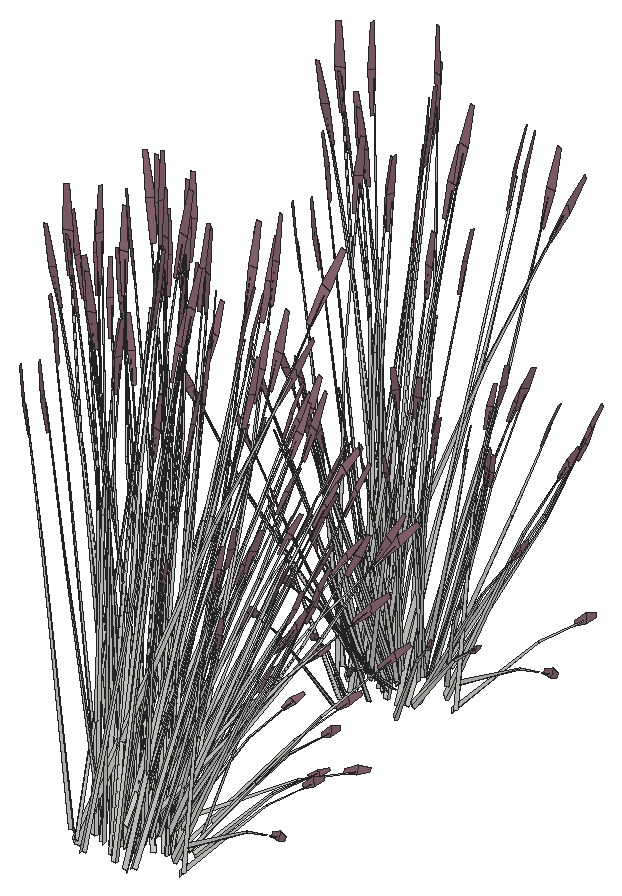
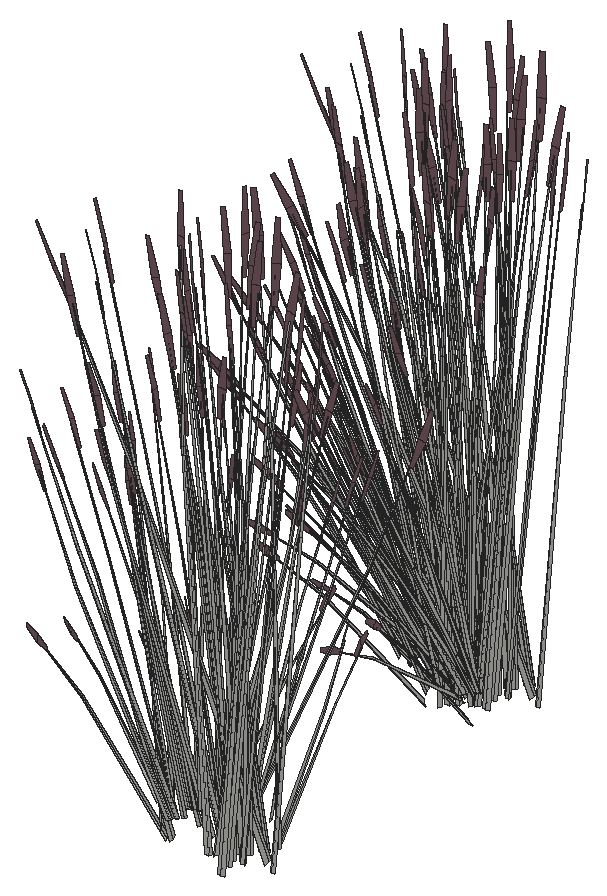
# SketchUp Ruby script. Lengths in inches.
U = 1.inch
M = Sketchup.active_model
def pt(a) = Geom::Point3d.new(a.map { |v| v * U })
def face(e, loops, mat)
  f = e.add_face(loops[0].map { |a| pt(a) })
  loops[1..].each { |l| e.add_face(l.map { |a| pt(a) }).erase! }
  f.material = f.back_material = mat if mat
  f
end
# faces: each face lists its corners as indices into pts; further lists are holes
def faces(e, pts, list, mat = nil) = list.each { |f| face(e, (f[0].is_a?(Array) ? f : [f]).map { |l| l.map { |i| pts[i] } }, mat) }
# xy, xz, yz: faces in a plane at the given z, y or x. An outline is a flat list of corners, or four numbers for a rectangle; further outlines are holes
def ring(l) = l.size == 4 ? [[l[0], l[1]], [l[2], l[1]], [l[2], l[3]], [l[0], l[3]]] : l.each_slice(2).to_a
def flat(e, list, mat, &to3) = list.each { |f| face(e, (f[0].is_a?(Array) ? f : [f]).map { |l| ring(l).map { |u, v| to3.(u, v) } }, mat) }
def xy(e, z, list, mat = nil) = flat(e, list, mat) { |x, y| [x, y, z] }
def xz(e, y, list, mat = nil) = flat(e, list, mat) { |x, z| [x, y, z] }
def yz(e, x, list, mat = nil) = flat(e, list, mat) { |y, z| [x, y, z] }
def lines(e, pts, list) = list.each { |a, b| e.add_line(pt(pts[a]), pt(pts[b])) }
# prism: a flat outline (further loops are holes) pulled along v
def prism(e, loops, v, mat = nil)
  f = face(e, loops, mat); d = Geom::Vector3d.new(v.map { |x| x * U })
  f.pushpull(f.normal.samedirection?(d) ? d.length : -d.length)
end
def box(e, o, s, mat = nil) = prism(e, [[o, [o[0] + s[0], o[1], o[2]], [o[0] + s[0], o[1] + s[1], o[2]], [o[0], o[1] + s[1], o[2]]]], [0, 0, s[2]], mat)
def at(x, y, z, deg = 0) = Geom::Transformation.translation(pt([x, y, z])) * Geom::Transformation.rotation(ORIGIN, Z_AXIS, deg.degrees)
def axes(o, x, y, z) = Geom::Transformation.new([*x, 0, *y, 0, *z, 0, *pt(o).to_a, 1])
def part(name) = M.definitions.add(name)
# library, detail: a bought-in or finely detailed component or shape, given as its bounding box
def library(name, o, s) = part(name).tap { |d| box(d.entities, o, s) }
def detail(e, o, s) = box(e.add_group.entities, o, s)
def put(e, d, t, mat = nil) = e.add_instance(d, t).tap { |i| i.material = mat if mat }
def group(e, t, mat = nil) = e.add_group.tap { |g| g.transformation = t; g.material = mat if mat }.entities
root = M.entities
M.materials.add("LightPink_Translucent").color = [144, 107, 117]
c1 = part("blade")
p = [[2.15,0.21,22],[0,0.17,0],[0.09,0.45,0],[2.18,0.31,22],[2.29,0.31,22],[0.38,0.45,0],
  [2.48,0.24,33],[2.49,0.24,33],[2.48,0.22,33]]
faces(c1.entities,p,[[0,1,2,3],[4,5,2,3],[6,3,4,7],[8,0,3,6]])
c2 = part("seeds")
p = [[0.3,-0.1,1.38],[-0.01,-0.03,1.59],[-0.01,-0.03,0.03],[0.14,-0.07,-0.07],[0.29,-0.03,3],[0.15,0.01,3.11]]
faces(c2.entities,p,[[0,1,2,3],[1,0,4,5]],"LightPink_Translucent")
c3 = part("blade with seeds")
put(c3.entities,c1,at(0,0,0))
put(c3.entities,c2,axes([2.4,0.25,30.99],[1.5799,-0.05474,1.17369],[-0.12525,1.92788,0.29478],[-0.07173,-0.02425,1.56792]))
put(root,c3,axes([70.95,556.1,39.31],[0.85545,-0.64616,-0.30978],[0.85545,0.64616,0.30978],[0,-0.20813,1.38974]))
put(root,c3,axes([70.95,592.55,38.96],[0.85545,-0.64616,-0.30978],[0.85545,0.64616,0.30978],[0,-0.20813,1.38974]))
put(root,c3,axes([74.82,588.375,39.0625],[-0.84686,0.59414,-0.03893],[-0.77596,-0.65071,-0.17649],[-0.05463,-0.18438,0.58215]))
put(root,c3,axes([74.48,557.78,39.64],[1.54892,0.2182,0.45755],[-0.31522,1.23236,0.17955],[-0.22636,-0.119,1.58856]))
put(root,c3,axes([74.48,594.23,39.3],[1.54892,0.2182,0.45755],[-0.31522,1.23236,0.17955],[-0.22636,-0.119,1.58856]))
put(root,c3,axes([74.08,557.5625,40],[-0.59459,0.93321,0.44739],[-1.23546,-0.44912,-0.21531],[0,-0.21512,1.43643]))
put(root,c3,axes([74.08,594.01,39.65],[-0.59459,0.93321,0.44739],[-1.23546,-0.44912,-0.21531],[0,-0.21512,1.43643]))
put(root,c3,axes([76.04,589.51,41.92],[-0.5849,-0.8421,-0.71045],[1.20401,-0.4693,0.08574],[-0.13677,-0.40688,1.00501]))
put(root,c3,axes([73.65,559.75,39.75],[1.31687,-0.27488,0.17642],[0.32517,1.02297,0.35086],[-0.11745,-0.14905,1.60407]))
put(root,c3,axes([73.65,596.2,39.41],[1.31687,-0.27488,0.17642],[0.32517,1.02297,0.35086],[-0.11745,-0.14905,1.60407]))
put(root,c3,axes([75.34,559.92,39.47],[-1.23546,-0.46496,0],[0.59459,-0.96613,0],[0,0,1.62707]))
put(root,c3,axes([76.27,589.64,41.99],[-0.36946,0.79643,0.35414],[-1.07787,-0.23229,-0.4572],[-0.09883,-0.32066,0.87481]))
put(root,c3,axes([78.2,561.08,39.65],[0.7662,1.03778,0],[-1.28187,0.57875,-0.51607],[-0.29196,0.13181,1.63711]))
put(root,c3,axes([74.3,561.53,42.34],[-1.20755,-0.27075,0.53283],[0.41292,-0.89013,0.43934],[0.07257,0.35005,1.10256]))
put(root,c3,axes([73.98,561.59,42.01],[-0.90301,0.35198,0.0643],[-0.44199,-0.64184,0.50621],[0.08721,0.28293,0.77189]))
put(root,c3,axes([77.5625,559.81,39.75],[0.35402,-1.02926,0.17642],[1.29548,0.29127,0.35086],[-0.22379,0.00501,1.60407]))
put(root,c3,axes([76.97,558.44,39.89],[0.90538,0.62224,0.1448],[-0.75521,0.70202,-0.41347],[-0.21021,0.09491,1.26744]))
put(root,c3,axes([76.64,557.68,39.58],[-1.1399,-0.8914,-0.06131],[1.1406,-0.89194,0],[-0.03981,-0.03113,1.75571]))
put(root,c3,axes([76.64,594.125,39.23],[-1.1399,-0.8914,-0.06131],[1.1406,-0.89194,0],[-0.03981,-0.03113,1.75571]))
put(root,c3,axes([76.94,557.99,40],[1.33077,-0.06393,0.44739],[0.12035,1.06125,-0.21531],[-0.23824,0.10756,1.43643]))
put(root,c3,axes([77.27,560.43,39.61],[1.53422,0.33662,0.30756],[-0.38383,1.20322,-0.36492],[-0.25393,0.15059,1.64885]))
put(root,c3,axes([75.03,587.65,38.43],[-0.20555,0.03731,1.76342],[-1.13672,-0.42002,-0.26939],[0.01907,-0.35034,0.30037]))
put(root,c3,axes([77.93,560.36,39.76],[1.14694,-0.51783,0.49651],[0.68554,0.92854,0],[-0.26122,0.11794,1.57504]))
put(root,c3,axes([76.15,588.8,41.46],[0.36946,-0.79643,-0.35414],[1.07787,0.23229,0.4572],[-0.09883,-0.32066,0.87481]))
put(root,c3,axes([74.34,556.65,39.64],[0.53281,1.15808,0.45755],[-1.52239,0.4027,0.17955],[0.01861,-0.2128,1.58856]))
put(root,c3,axes([74.34,593.1,39.3],[0.53281,1.15808,0.45755],[-1.52239,0.4027,0.17955],[0.01861,-0.2128,1.58856]))
put(root,c3,axes([74.1,556.5,39.49],[0.59459,-0.93321,-0.44739],[1.23546,0.44912,0.21531],[0,-0.21512,1.43643]))
put(root,c3,axes([74.1,592.95,39.15],[0.59459,-0.93321,-0.44739],[1.23546,0.44912,0.21531],[0,-0.21512,1.43643]))
put(root,c3,axes([75.62,559.51,39.48],[-0.39985,-0.89288,0],[1.1418,-0.31268,0],[0,0,1.54371]))
put(root,c3,axes([74.17,561.4,38.77],[0.19833,-0.05635,1.76342],[1.19302,0.31018,-0.26939],[0.03489,0.3496,0.30037]))
put(root,c3,axes([74.43,561.71,41.8],[-0.36946,0.79643,-0.35414],[-1.07787,-0.23229,0.4572],[0.09883,0.32066,0.87481]))
put(root,c3,axes([77.24,557.75,39.49],[-0.59459,0.93321,-0.44739],[-1.23546,-0.44912,0.21531],[0,0.21512,1.43643]))
put(root,c3,axes([76.6,588.92,41.67],[0.90301,-0.35198,0.0643],[0.44199,0.64184,0.50621],[-0.08721,-0.28293,0.77189]))
put(root,c3,axes([73.67,563.12,41.99],[0.15534,0.16677,1.74944],[1.25362,0.06552,-0.27667],[0.12606,0.3678,0.14031]))
put(root,c3,axes([79.59,557.18,39.75],[-0.96285,-0.75439,0.17642],[0.97031,-0.7317,0.35086],[-0.10634,0.15406,1.60407]))
put(root,c3,axes([76.26,556.75,39.48],[0,-1.19833,0],[1.53239,0,0],[0,0,1.79456]))
put(root,c3,axes([76.26,593.2,39.14],[0,-1.19833,0],[1.53239,0,0],[0,0,1.79456]))
put(root,c3,axes([76.28,588.98,41.67],[1.20755,0.27075,0.48003],[-0.41292,0.89013,0.3958],[-0.07257,-0.35005,0.9933]))
put(root,c3,axes([74.84,556.97,39.71],[1.3808,0.50196,0.24065],[-0.66454,1.04299,0.50002],[0,-0.24043,1.60543]))
put(root,c3,axes([74.84,593.42,39.37],[1.3808,0.50196,0.24065],[-0.66454,1.04299,0.50002],[0,-0.24043,1.60543]))
put(root,c3,axes([77.03,557.23,39.57],[0,1.19774,-0.05637],[-1.53239,0,0],[0,0.03764,1.79368]))
put(root,c3,axes([74.39,556.27,40],[-1.33077,0.06393,0.44739],[-0.12035,-1.06125,-0.21531],[0.23824,-0.10756,1.43643]))
put(root,c3,axes([74.39,592.72,39.65],[-1.33077,0.06393,0.44739],[-0.12035,-1.06125,-0.21531],[0.23824,-0.10756,1.43643]))
put(root,c3,axes([74.3125,560.87,42.33],[0.36946,-0.79643,0.35414],[1.07787,0.23229,-0.4572],[0.09883,0.32066,0.87481]))
put(root,c3,axes([73.77,554.45,39.75],[-0.35402,1.02926,0.17642],[-1.29548,-0.29127,0.35086],[0.22379,-0.00501,1.60407]))
put(root,c3,axes([73.77,590.89,39.41],[-0.35402,1.02926,0.17642],[-1.29548,-0.29127,0.35086],[0.22379,-0.00501,1.60407]))
put(root,c3,axes([76.3,559.54,39.57],[0.53281,1.18979,-0.06012],[-1.52239,0.41691,0],[0.01861,0.04155,1.72173]))
put(root,c3,axes([73.14,589.625,39.31],[-0.7662,-1.03778,0],[1.28187,-0.57875,-0.51607],[0.29196,-0.13181,1.63711]))
put(root,c3,axes([74.54,561,42.26],[0.5849,0.8421,-0.71045],[-1.20401,0.4693,0.08574],[0.13677,0.40688,1.00501]))
put(root,c3,axes([80.7,557.98,39.48],[-1.53164,-0.00828,-0.04976],[0,-1.1575,0.49943],[-0.04813,0.2635,1.58352]))
put(root,c3,axes([77.6875,554.5,39.75],[-1.31687,0.27488,0.17642],[-0.32517,-1.02297,0.35086],[0.11745,0.14905,1.60407]))
put(root,c3,axes([77.6875,590.95,39.41],[-1.31687,0.27488,0.17642],[-0.32517,-1.02297,0.35086],[0.11745,0.14905,1.60407]))
put(root,c3,axes([76.34,587.12,39.7],[0.15721,0.60392,1.1486],[-0.87211,-0.33448,0.84392],[0.09385,-0.30923,0.25299]))
put(root,c3,axes([75.76,563.71,42.92],[0.84686,-0.59414,-0.06488],[0.77596,0.65071,-0.29416],[0.05463,0.18438,0.97024]))
put(root,c3,axes([75.53,555.99,39.64],[-1.01611,0.93987,0.45755],[-1.20717,-0.82966,0.17955],[0.24496,-0.0938,1.58856]))
put(root,c3,axes([75.53,592.44,39.3],[-1.01611,0.93987,0.45755],[-1.20717,-0.82966,0.17955],[0.24496,-0.0938,1.58856]))
put(root,c3,axes([77.27,557.48,39.49],[0.85545,0.66896,0],[-0.85545,0.66896,0],[0,0,1.69266]))
put(root,c3,axes([77.26,556.69,40],[0.59459,-0.93321,0.44739],[1.23546,0.44912,-0.21531],[0,0.21512,1.43643]))
put(root,c3,axes([76.74,559.93,39.48],[1.23546,0.46496,0],[-0.59459,0.96613,0],[0,0,1.74954]))
put(root,c3,axes([74.98,561.17,41.96],[1.20468,0.25962,-0.51099],[-0.41292,0.89013,-0.3958],[0.11046,0.35838,0.97773]))
put(root,c3,axes([73.95,561.21,42.3125],[1.19922,-0.48218,-0.1216],[0.58932,0.85579,-0.67495],[0.15822,0.36063,1.02557]))
put(root,c3,axes([76.86,556.47,39.66],[-1.54892,-0.2182,0.49198],[0.31522,-1.23236,0.19306],[0.22636,0.119,1.70813]))
put(root,c3,axes([80.08,588.1,41.64],[-0.12446,0.07911,1.77383],[-1.21937,-0.26689,-0.16761],[-0.04414,-0.34521,0.31391]))
put(root,c3,axes([79.12,590.39,41.97],[-1.34686,-0.05131,-0.1216],[0.03681,-0.97156,-0.67495],[0.09356,-0.37418,1.02557]))
put(root,c3,axes([80.38,558.15,39.31],[-0.85545,0.64616,-0.30978],[-0.85545,-0.64616,0.30978],[0,0.20813,1.38974]))
put(root,c3,axes([77.94,558.03,39.37],[0.44936,0.94823,-0.69212],[-1.29441,0.3415,-0.18165],[0.04967,0.32109,1.52773]))
put(root,c3,axes([77.3,557.02,39.48],[1.37109,0,0],[0,1.07219,0],[0,0,1.78407]))
put(root,c3,axes([77.3,593.46,39.14],[1.37109,0,0],[0,1.07219,0],[0,0,1.78407]))
put(root,c3,axes([78.59,590.54,41.99],[-0.82919,0.54528,0.35414],[-0.78493,-0.62262,-0.4572],[0.11943,-0.31634,0.87481]))
put(root,c3,axes([75.98,555.83,40],[-0.73619,-0.86927,0.44739],[1.11511,-0.61213,-0.21531],[0.23824,0.10756,1.43643]))
put(root,c3,axes([75.98,592.28,39.65],[-0.73619,-0.86927,0.44739],[1.11511,-0.61213,-0.21531],[0.23824,0.10756,1.43643]))
put(root,c3,axes([74.64,556.04,39.94],[-0.1428,-1.18174,-0.29095],[1.48733,-0.07145,-0.50002],[0.26191,-0.15741,1.59708]))
put(root,c3,axes([74.64,592.49,39.6],[-0.1428,-1.18174,-0.29095],[1.48733,-0.07145,-0.50002],[0.26191,-0.15741,1.59708]))
put(root,c3,axes([77.77,556.91,39.89],[1.1418,-0.30203,0.1448],[0.39985,0.86246,-0.41347],[0,0.18981,1.26744]))
put(root,c3,axes([78.2,590.02,41.62],[-0.87728,-0.69587,-0.51099],[0.92674,-0.60943,-0.3958],[0.13348,-0.35356,0.97773]))
put(root,c3,axes([77.38,556.98,39.94],[1.38012,0.49416,-0.29095],[-0.66454,1.04299,-0.50002],[0.04337,0.25608,1.59708]))
put(root,c3,axes([74.45,553.42,39.31],[1.14332,0.25625,-0.30978],[-0.28787,0.90242,0.30978],[0.23049,-0.10406,1.38974]))
put(root,c3,axes([74.45,589.87,38.96],[1.14332,0.25625,-0.30978],[-0.28787,0.90242,0.30978],[0.23049,-0.10406,1.38974]))
put(root,c3,axes([77.625,588.78,39.53],[-0.34835,0.20963,1.43002],[-1.04325,-0.36691,-0.30754],[0.19338,-0.4563,0.61141]))
put(root,c3,axes([80.38,557.21,39.76],[0,-1.03566,0.49651],[1.37109,0,0],[0,0.23588,1.57504]))
put(root,c3,axes([80.97,558.17,39.3],[0,1.03566,-0.49651],[-1.37109,0,0],[0,0.23588,1.57504]))
put(root,c3,axes([77.31,561.3125,42.01],[-1.21888,0.23767,0.48003],[-0.21154,-0.93233,0.3958],[0.28666,0.27478,0.9933]))
put(root,c3,axes([74.18,589.46,38.95],[1.14694,-0.51783,-0.49651],[0.68554,0.92854,0],[0.26122,-0.11794,1.57504]))
put(root,c3,axes([77.07,561.5,42.01],[-0.55698,0.6579,0.0643],[-0.79316,-0.38303,0.50621],[0.25643,0.21093,0.77189]))
put(root,c3,axes([75.66,559.33,41.15],[-0.28013,-0.33252,1.71376],[1.29445,-0.27994,0.13857],[0.29256,0.52202,0.73262]))
put(root,c3,axes([76.48,555.59,39.89],[0.23642,-0.92427,0.1448],[1.15506,0.16044,-0.41347],[0.21021,0.09491,1.26744]))
put(root,c3,axes([76.48,592.04,39.55],[0.23642,-0.92427,0.1448],[1.15506,0.16044,-0.41347],[0.21021,0.09491,1.26744]))
put(root,c3,axes([78.12,553.98,39.76],[-1.14694,-0.51783,0.49651],[0.68554,-0.92854,0],[0.26122,0.11794,1.57504]))
put(root,c3,axes([78.12,590.43,39.41],[-1.14694,-0.51783,0.49651],[0.68554,-0.92854,0],[0.26122,0.11794,1.57504]))
put(root,c3,axes([78.47,590.34,41.92],[0.03189,-0.95798,-0.71045],[1.34277,0.06434,0.08574],[0.14171,-0.40585,1.00501]))
put(root,c3,axes([77.12,559.39,39.46],[1.2866,-0.3514,-0.19198],[0.45209,1.01223,0.00008],[0.14202,-0.03884,1.73897]))
put(root,c3,axes([76.9,560.74,42.33],[-0.18927,-0.83419,0.35414],[1.08199,-0.22027,-0.4572],[0.29062,0.23905,0.87481]))
put(root,c3,axes([77.14,556.38,39.49],[0.73619,0.86927,-0.44739],[-1.11511,0.61213,0.21531],[0.23824,0.10756,1.43643]))
put(root,c3,axes([77.63,555.94,41.75],[-1.05895,-0.53811,1.38283],[1.11816,-0.83781,0.59665],[0.34166,0.5049,1.33663]))
put(root,c3,axes([79.03,589.76,41.46],[0.82919,-0.54528,-0.35414],[0.78493,0.62262,0.4572],[0.11943,-0.31634,0.87481]))
put(root,c3,axes([75.85,561.91,41.99],[0.00363,-0.12539,1.77383],[1.0502,-0.55319,-0.16761],[0.36479,0.19745,0.31391]))
put(root,c3,axes([79.35,590.04,41.67],[1.00708,0.04826,0.0643],[-0.02761,0.72867,0.50621],[0.10538,-0.27912,0.77189]))
put(root,c3,axes([79.23,560.32,40.04],[-0.69001,-0.29779,1.1486],[0.89096,-0.30257,0.84392],[0.24031,0.2563,0.25299]))
put(root,c3,axes([76.77,560.01,39.87],[0.02163,-0.34331,1.43002],[1.03345,-0.38348,-0.30754],[0.31903,0.4109,0.61141]))
put(root,c3,axes([80.35,588.84,41.65],[-0.01183,-0.20612,1.74944],[-0.99913,-0.59572,-0.27667],[0.15447,-0.36112,0.14031]))
put(root,c3,axes([75.54,591.59,38.99],[0.82544,-0.77843,-0.62353],[1.0254,0.70586,-0.16365],[0.33076,-0.19418,1.37633]))
put(root,c3,axes([79.02,589.97,41.67],[0.87265,0.70663,0.48003],[-0.92674,0.60943,0.3958],[0.16097,-0.33153,0.9933]))
put(root,c3,axes([79.16,554.45,39.31],[0.28787,0.90242,-0.30978],[-1.14332,0.25625,0.30978],[0.23049,0.10406,1.38974]))
put(root,c3,axes([81.31,557.39,39.65],[1.53239,0,0],[0,1.1575,-0.51607],[0,0.26363,1.63711]))
put(root,c3,axes([76.36,555.89,39.94],[1.23732,-0.68758,-0.29095],[0.8228,0.97154,-0.50002],[0.30528,0.09867,1.59708]))
put(root,c3,axes([76.36,592.34,39.6],[1.23732,-0.68758,-0.29095],[0.8228,0.97154,-0.50002],[0.30528,0.09867,1.59708]))
put(root,c3,axes([79.34,561.68,39.95],[-0.78586,-0.03248,1.0506],[0.51898,-0.68985,0.58006],[0.31045,0.24509,0.8241]))
put(root,c3,axes([80.03,555.77,42.33],[-1.06674,0.14801,0.35414],[-0.28168,-0.84611,-0.4572],[0.30569,-0.22726,0.87481]))
put(root,c3,axes([80.03,592.22,41.99],[-1.06674,0.14801,0.35414],[-0.28168,-0.84611,-0.4572],[0.30569,-0.22726,0.87481]))
put(root,c3,axes([76.96,589.85,40.8125],[-0.22818,0.35597,1.71376],[-0.95725,-0.73667,0.13857],[0.43183,-0.45914,0.73262]))
put(root,c3,axes([76.8,561.17,42.3125],[0.73026,-0.88648,-0.1216],[1.05755,0.51071,-0.67495],[0.36761,0.25045,1.02557]))
put(root,c3,axes([73.23,555.28,38.87],[-1.20625,0.41464,1.28929],[-0.38394,-1.1897,0.50096],[0.74071,0.01979,1.46642]))
put(root,c3,axes([73.23,591.73,38.53],[-1.20625,0.41464,1.28929],[-0.38394,-1.1897,0.50096],[0.74071,0.01979,1.46642]))
put(root,c3,axes([80.59,592.3,41.97],[-1.1336,-0.57106,-0.1216],[0.65308,-0.827,-0.67495],[0.32027,-0.28747,1.02557]))
put(root,c3,axes([77.67,560.73,41.96],[1.20928,-0.24619,-0.51099],[0.21154,0.93233,-0.3958],[0.32481,0.26718,0.97773]))
put(root,c3,axes([78.78,553.4375,39.65],[0.7662,-1.03778,0],[1.28187,0.57875,-0.51607],[0.29196,0.13181,1.63711]))
put(root,c3,axes([78.78,589.89,39.3125],[0.7662,-1.03778,0],[1.28187,0.57875,-0.51607],[0.29196,0.13181,1.63711]))
put(root,c3,axes([80.0625,589.43,38.43],[-0.18342,-0.08159,1.76342],[-0.47115,-0.9115,-0.26939],[0.31784,-0.24736,0.30037]))
put(root,c3,axes([79.06,559.61,42.33],[-0.69728,-0.64842,0.35414],[0.79619,-0.61382,-0.4572],[0.40453,0.09339,0.87481]))
put(root,c3,axes([79.48,554.0625,39.3],[1.14694,0.51783,-0.49651],[-0.68554,0.92854,0],[0.26122,0.11794,1.57504]))
put(root,c3,axes([79.48,590.51,38.95],[1.14694,0.51783,-0.49651],[-0.68554,0.92854,0],[0.26122,0.11794,1.57504]))
put(root,c3,axes([79.6875,560.2,42.01],[-0.06171,0.78753,0.0643],[-0.9318,-0.02159,0.50621],[0.35694,0.08241,0.77189]))
put(root,c3,axes([79.42,561.43,38.77],[0.08928,-0.14952,1.76342],[1.12407,-0.44035,-0.26939],[0.34078,0.22791,0.30037]))
put(root,c3,axes([79.77,559.95,42.01],[-0.90362,0.68241,0.48003],[-0.77932,-0.72471,0.3958],[0.42395,0.12588,0.9933]))
put(root,c3,axes([80.02,591.62,41.62],[-0.31482,-0.94565,-0.51099],[1.19224,-0.16542,-0.3958],[0.34166,-0.254,0.97773]))
put(root,c3,axes([82.12,560.05,41.21],[-0.23455,-0.87059,-0.03492],[1.10861,-0.20015,-0.15832],[0.23151,0.05519,0.52218]))
put(root,c3,axes([80.2,557.8,42.33],[-1.01846,-0.28891,0.35414],[0.29705,-0.84289,-0.4572],[0.41005,-0.07729,0.87481]))
put(root,c3,axes([80.2,594.24,41.99],[-1.01846,-0.28891,0.35414],[0.29705,-0.84289,-0.4572],[0.41005,-0.07729,0.87481]))
put(root,c3,axes([77.8,556.04,39.34],[1.27479,0.1698,-0.62353],[-0.26901,1.04736,-0.16365],[0.38043,0.12691,1.37633]))
put(root,c3,axes([83.23,556.66,39.54],[-0.75977,-0.66224,-0.06488],[0.83212,-0.6068,-0.29416],[0.23578,-0.04272,0.97024]))
put(root,c3,axes([83.23,593.11,39.2],[-0.75977,-0.66224,-0.06488],[0.83212,-0.6068,-0.29416],[0.23578,-0.04272,0.97024]))
put(root,c3,axes([81.49,589.74,39.7],[-0.40819,0.5272,1.1486],[-0.35086,-0.70831,0.84392],[0.33713,-0.17749,0.25299]))
put(root,c3,axes([81,555.64,42.01],[0.8413,0.43556,0.0643],[-0.48981,0.62025,0.50621],[0.26973,-0.20053,0.77189]))
put(root,c3,axes([81,592.09,41.67],[0.8413,0.43556,0.0643],[-0.48981,0.62025,0.50621],[0.26973,-0.20053,0.77189]))
put(root,c3,axes([80.77,555.45,42.01],[0.30393,0.95317,0.48003],[-1.19224,0.16542,0.3958],[0.35138,-0.22417,0.9933]))
put(root,c3,axes([80.77,591.9,41.67],[0.30393,0.95317,0.48003],[-1.19224,0.16542,0.3958],[0.35138,-0.22417,0.9933]))
put(root,c3,axes([77.54,558.29,41.15],[-0.45521,-0.17844,1.71376],[0.94204,-0.74856,0.13857],[0.58713,0.33769,0.73262]))
put(root,c3,axes([83.38,592.05,41.64],[-0.16006,-0.00787,1.77383],[-0.66468,-0.8428,-0.16761],[0.26693,-0.27711,0.31391]))
put(root,c3,axes([80.9,591.72,41.46],[1.06674,-0.14801,-0.35414],[0.28168,0.84611,0.4572],[0.30569,-0.22726,0.87481]))
put(root,c3,axes([80.06,592,41.92],[0.64013,-0.81717,-0.71045],[1.12174,0.58074,0.08574],[0.38221,-0.29607,1.00501]))
put(root,c3,axes([81.125,558.06,42.01],[0.4501,0.70615,0.0643],[-0.82077,0.34564,0.50621],[0.36181,-0.0682,0.77189]))
put(root,c3,axes([80.05,559.95,41.8],[0.69728,0.64842,-0.35414],[-0.79619,0.61382,0.4572],[0.40453,0.09339,0.87481]))
put(root,c3,axes([79.25,560.03,42.3125],[0.06562,-1.05324,-0.1216],[1.2424,0.02879,-0.67495],[0.4785,0.07316,1.02557]))
put(root,c3,axes([80.63,558.08,42.3125],[-0.6166,-0.93779,-0.1216],[1.09436,-0.46085,-0.67495],[0.46117,-0.12373,1.02557]))
put(root,c3,axes([80.63,594.53,41.97],[-0.6166,-0.93779,-0.1216],[1.09436,-0.46085,-0.67495],[0.46117,-0.12373,1.02557]))
put(root,c3,axes([81.04,557.81,42.01],[-0.34623,0.9443,0.48003],[-1.13828,-0.3229,0.3958],[0.44763,-0.05675,0.9933]))
put(root,c3,axes([80.33,559.39,41.99],[0.26289,-0.01751,1.74944],[0.72108,-0.8046,-0.27667],[0.46761,0.10621,0.14031]))
put(root,c3,axes([80.58,557.27,41.96],[0.332,-0.94205,-0.51099],[1.13828,0.3229,-0.3958],[0.45829,-0.08638,0.97773]))
put(root,c3,axes([80.58,593.72,41.62],[0.332,-0.94205,-0.51099],[1.13828,0.3229,-0.3958],[0.45829,-0.08638,0.97773]))
put(root,c3,axes([83.4375,557.875,40.04],[-0.75718,0.17097,1.1486],[0.35641,-0.70661,0.84392],[0.40168,0.04835,0.25299]))
put(root,c3,axes([80.98,591.25,39.53],[-0.4378,-0.03068,1.43002],[-0.44851,-0.8229,-0.30754],[0.53783,-0.23279,0.61141]))
put(root,c3,axes([81.28,557.7,41.8],[1.01846,0.28891,-0.35414],[-0.29705,0.84289,0.4572],[0.41005,-0.07729,0.87481]))
put(root,c3,axes([81.28,594.15,41.46],[1.01846,0.28891,-0.35414],[-0.29705,0.84289,0.4572],[0.41005,-0.07729,0.87481]))
put(root,c3,axes([79.31,559.52,42.26],[1.22504,0.02494,-0.71045],[-0.08228,1.05005,0.08574],[0.51899,0.11081,1.00501]))
put(root,c3,axes([81.79,557.54,39.26],[-0.7893,0.12429,1.41583],[-0.12563,-0.9893,0.08104],[0.55282,-0.14974,0.80566]))
put(root,c3,axes([81.79,593.99,38.92],[-0.7893,0.12429,1.41583],[-0.12563,-0.9893,0.08104],[0.55282,-0.14974,0.80566]))
put(root,c3,axes([82.66,556.89,38.77],[-0.06405,-0.15723,1.76342],[0.44421,-0.91974,-0.26939],[0.4481,-0.01323,0.30037]))
put(root,c3,axes([82.66,593.34,38.43],[-0.06405,-0.15723,1.76342],[0.44421,-0.91974,-0.26939],[0.4481,-0.01323,0.30037]))
put(root,c3,axes([83.08,560.86,41.99],[-0.11081,-0.09067,1.77383],[0.2424,-0.97188,-0.16761],[0.43649,-0.06209,0.31391]))
put(root,c3,axes([78.5,556.66,41.15],[-0.50831,0.02346,1.71376],[0.33721,-1.01661,0.13857],[0.72439,0.06288,0.73262]))
put(root,c3,axes([80.36,557.62,42.26],[1.07686,-0.45739,-0.71045],[0.60013,0.94154,0.08574],[0.52031,-0.10696,1.00501]))
put(root,c3,axes([80.36,594.0625,41.92],[1.07686,-0.45739,-0.71045],[0.60013,0.94154,0.08574],[0.52031,-0.10696,1.00501]))
put(root,c3,axes([83.98,556.61,41.99],[0.17006,-0.15775,1.74944],[-0.21766,-0.96766,-0.27667],[0.42669,-0.18347,0.14031]))
put(root,c3,axes([83.98,593.06,41.65],[0.17006,-0.15775,1.74944],[-0.21766,-0.96766,-0.27667],[0.42669,-0.18347,0.14031]))
put(root,c3,axes([82.02,559.01,39.87],[-0.29514,-0.25472,1.43002],[0.38401,-0.84262,-0.30754],[0.59714,0.11414,0.61141]))
